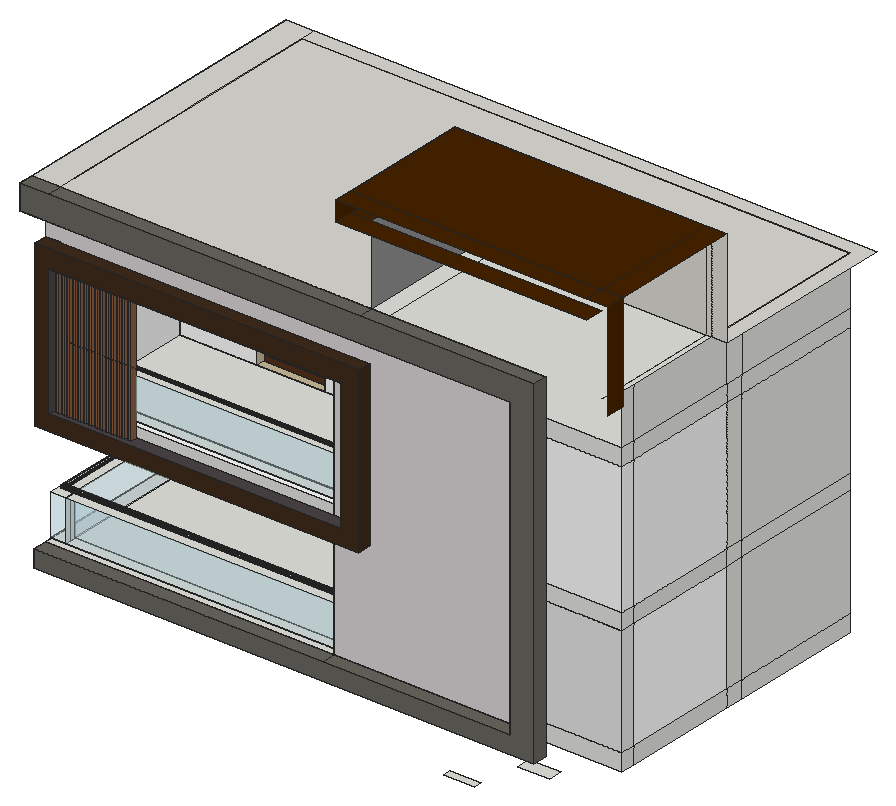
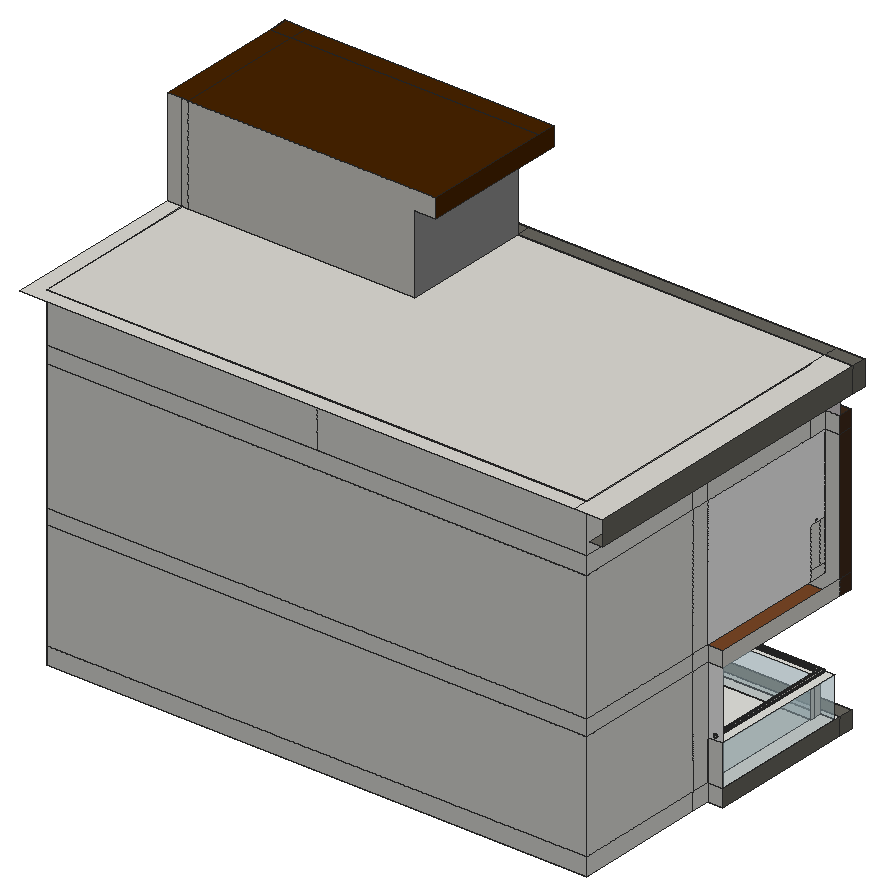
# SketchUp Ruby script. Lengths in inches.
U = 1.inch
M = Sketchup.active_model
def pt(a) = Geom::Point3d.new(a.map { |v| v * U })
def face(e, loops, mat)
  f = e.add_face(loops[0].map { |a| pt(a) })
  loops[1..].each { |l| e.add_face(l.map { |a| pt(a) }).erase! }
  f.material = f.back_material = mat if mat
  f
end
# faces: each face lists its corners as indices into pts; further lists are holes
def faces(e, pts, list, mat = nil) = list.each { |f| face(e, (f[0].is_a?(Array) ? f : [f]).map { |l| l.map { |i| pts[i] } }, mat) }
# xy, xz, yz: faces in a plane at the given z, y or x. An outline is a flat list of corners, or four numbers for a rectangle; further outlines are holes
def ring(l) = l.size == 4 ? [[l[0], l[1]], [l[2], l[1]], [l[2], l[3]], [l[0], l[3]]] : l.each_slice(2).to_a
def flat(e, list, mat, &to3) = list.each { |f| face(e, (f[0].is_a?(Array) ? f : [f]).map { |l| ring(l).map { |u, v| to3.(u, v) } }, mat) }
def xy(e, z, list, mat = nil) = flat(e, list, mat) { |x, y| [x, y, z] }
def xz(e, y, list, mat = nil) = flat(e, list, mat) { |x, z| [x, y, z] }
def yz(e, x, list, mat = nil) = flat(e, list, mat) { |y, z| [x, y, z] }
def lines(e, pts, list) = list.each { |a, b| e.add_line(pt(pts[a]), pt(pts[b])) }
# prism: a flat outline (further loops are holes) pulled along v
def prism(e, loops, v, mat = nil)
  f = face(e, loops, mat); d = Geom::Vector3d.new(v.map { |x| x * U })
  f.pushpull(f.normal.samedirection?(d) ? d.length : -d.length)
end
def box(e, o, s, mat = nil) = prism(e, [[o, [o[0] + s[0], o[1], o[2]], [o[0] + s[0], o[1] + s[1], o[2]], [o[0], o[1] + s[1], o[2]]]], [0, 0, s[2]], mat)
def at(x, y, z, deg = 0) = Geom::Transformation.translation(pt([x, y, z])) * Geom::Transformation.rotation(ORIGIN, Z_AXIS, deg.degrees)
def axes(o, x, y, z) = Geom::Transformation.new([*x, 0, *y, 0, *z, 0, *pt(o).to_a, 1])
def part(name) = M.definitions.add(name)
# library, detail: a bought-in or finely detailed component or shape, given as its bounding box
def library(name, o, s) = part(name).tap { |d| box(d.entities, o, s) }
def detail(e, o, s) = box(e.add_group.entities, o, s)
def put(e, d, t, mat = nil) = e.add_instance(d, t).tap { |i| i.material = mat if mat }
def group(e, t, mat = nil) = e.add_group.tap { |g| g.transformation = t; g.material = mat if mat }.entities
root = M.entities
M.materials.add("[Asphalt New]").color = [76, 68, 70]
M.materials.add("[Blinds Cellular White]").color = [217, 211, 213]
M.materials.add("[Blinds Cellular White]1").color = [217, 211, 213]
M.materials.add("[Carrera Marble]").color = [252, 252, 252]
M.materials.add("[Carrera Marble]1").color = [247, 247, 247]
M.materials.add("[Color C08]").color = [71, 35, 0]
M.materials.add("[Color M01]").color = [226, 226, 226]
M.materials.add("[Color M02]").color = [198, 198, 198]
M.materials.add("[Color M04]").color = [142, 142, 142]
M.materials.add("[Formica Graystone]").color = [104, 102, 94]
M.materials.add("[Quartz Light Brown]").color = [199, 184, 152]
M.materials.add("[Quartz Light Grey]").color = [251, 251, 252]
M.materials.add("[Sandstone]").color = [63, 43, 28]
M.materials.add("[Terrazzo Tile Light]").color = [219, 217, 210]
M.materials.add("[Translucent Glass Safety]").color = [213, 245, 255]
M.materials["[Translucent Glass Safety]"].alpha = 0.35
M.materials.add("[Wood Bamboo]").color = [168, 99, 40]
M.materials.add("[Wood Floor Light]").color = [181, 156, 112]
M.materials.add("[Wood Veneer 01]").color = [84, 49, 25]
M.materials.add("[Wood Veneer 01]1").color = [120, 70, 37]
M.materials.add("[Wood Veneer 02]").color = [140, 94, 67]
xy(root,348.79,[[480.71,442.77,510.46,449.52]])
xy(root,380.34,[[551.08,442.77,580.83,455.77]])
xy(root,382.42,[[190.84,583.41,253.72,588.28]],"[Quartz Light Brown]")
xy(root,382.71,[[295.95,583.41,360.57,591.84]],"[Quartz Light Brown]")
xy(root,397.48,[[118.15,583.41,635.5,601.39],[118.15,601.39,635.5,728.625]])
xy(root,397.48,[[104.01,429.02,376.83,442.77],[376.83,429.02,577.15,442.77]],"[Formica Graystone]")
xy(root,397.48,[[104.01,442.77,104.01,583.41,635.5,583.41,635.5,460.01,376.83,460.01,376.83,442.77]],"[Wood Veneer 01]1")
xy(root,413.92,[[104.01,442.77,376.83,449.27],[104.01,449.27,118.15,583.41],[118.15,449.27,376.83,460.01],[118.15,460.01,635.5,583.41],[118.15,583.41,118.15,601.39,635.5,601.39,635.5,583.41,258.21,583.41,258.21,589.78,192.46,589.78,192.46,583.41],
  [118.15,601.39,635.5,728.625]])
xy(root,413.92,[[104.01,429.02,376.83,442.77],[376.83,429.02,553.9,442.77]],"[Formica Graystone]")
xy(root,413.92,[[192.46,583.41,258.21,589.78]],"[Quartz Light Brown]")
xy(root,434.25,[[289.17,583.41,357.54,594.28]],"[Quartz Light Brown]")
xy(root,452.92,[[104.01,449.27,118.15,583.41],[118.15,449.27,376.83,460.01]])
xy(root,498.23,[[192.46,583.41,258.21,589.78]],"[Quartz Light Brown]")
xy(root,502.625,[[289.17,583.41,357.54,594.28]],"[Quartz Light Brown]")
xy(root,517.48,[[118.15,583.41,635.5,601.39],[118.15,601.39,635.5,728.625]])
xy(root,517.48,[[104.01,429.65,410.58,442.77]],"[Asphalt New]")
xy(root,517.48,[[104.01,442.77,104.01,583.41,635.5,583.41,635.5,460.01,376.83,460.01,376.83,442.77]],"[Wood Veneer 01]1")
xy(root,532.23,[[119.9375,435.4,123.02,441.08],[125.125,435.4,128.2,441.08],[130.3125,435.4,133.39,441.08],[135.5,435.4,138.58,441.08],[140.6875,435.4,143.77,441.08],
  [145.875,435.4,148.95,441.08],[151.0625,435.4,154.14,441.08],[156.25,435.4,159.33,441.08],[161.4375,435.4,164.52,441.08],[166.625,435.4,169.7,441.08],
  [171.8125,435.4,174.89,441.08],[177,435.4,180.08,441.08],[182.1875,435.4,185.27,441.08],[187.375,435.4,190.45,441.08],[118.15,442.77,376.83,460.01],
  [118.15,460.01,635.5,583.41],[118.15,583.41,118.15,601.39,635.5,601.39,635.5,583.41,255.91,583.41,255.91,590.97,191.73,590.97,191.73,583.41],[118.15,601.39,635.5,728.625]])
xy(root,532.23,[[[118.15,429.65,393.7,442.77],[119.9375,435.4,123.02,441.08],[125.125,435.4,128.2,441.08],[130.3125,435.4,133.39,441.08],[135.5,435.4,138.58,441.08],[140.6875,435.4,143.77,441.08],[145.875,435.4,148.95,441.08],[151.0625,435.4,154.14,441.08],[156.25,435.4,159.33,441.08],[161.4375,435.4,164.52,441.08],[166.625,435.4,169.7,441.08],[171.8125,435.4,174.89,441.08],[177,435.4,180.08,441.08],[182.1875,435.4,185.27,441.08],[187.375,435.4,190.45,441.08]]],"[Asphalt New]")
xy(root,532.23,[[191.73,583.41,255.91,590.97]],"[Quartz Light Brown]")
xy(root,553.27,[[286.83,583.41,353,594.78]],"[Quartz Light Brown]")
xy(root,631.6,[[191.73,583.41,255.91,590.97]],"[Quartz Light Brown]")
xy(root,633.96,[[286.83,583.41,353,594.78]],"[Quartz Light Brown]")
xy(root,655.42,[[119.9375,435.4,123.02,441.08]])
xy(root,655.79,[[118.15,583.41,635.5,601.39],[118.15,601.39,635.5,728.625]])
xy(root,655.79,[[[118.15,429.65,118.15,583.41,635.5,583.41,635.5,460.01,376.83,460.01,376.83,442.77,393.7,442.77,393.7,429.65],[125.125,435.4,128.2,441.08],[130.3125,435.4,133.39,441.08],[135.5,435.4,138.58,441.08],[140.6875,435.4,143.77,441.08],[145.875,435.4,148.95,441.08],[151.0625,435.4,154.14,441.08],[156.25,435.4,159.33,441.08],[161.4375,435.4,164.52,441.08],[166.625,435.4,169.7,441.08],[171.8125,435.4,174.89,441.08],[177,435.4,180.08,441.08],[182.1875,435.4,185.27,441.08],[187.375,435.4,190.45,441.08]]],"[Wood Veneer 01]1")
xy(root,672.23,[[118.15,442.77,376.83,728.625],[376.83,460.01,635.5,728.625]])
xy(root,672.23,[[104.01,429.65,410.58,442.77]],"[Sandstone]")
xy(root,695.82,[[91.26,429.02,118.15,442.77],[118.15,429.02,553.9,442.77],[91.26,442.77,104.01,742.77]],"[Formica Graystone]")
xy(root,719.42,[[91.26,429.02,118.15,442.77],[118.15,429.02,412.79,442.77],[412.79,429.02,577.15,442.77]],"[Formica Graystone]")
xy(root,719.42,[[91.26,442.77,118.15,742.77],[118.15,442.77,412.79,442.77,412.79,566.02,635.5,566.02,635.5,728.625,118.15,728.625],[635.5,566.02,649.65,566.02,649.65,742.77,118.15,742.77,118.15,728.625,635.5,728.625]],"[Terrazzo Tile Light]")
xy(root,793.89,[[392.48,424.96,630.01,442.77],[392.48,442.77,412.79,566.02]],"[Color C08]")
xy(root,812.1,[[630.01,424.96,649.65,442.77],[630.01,442.77,649.65,566.02]],"[Color C08]")
xz(root,429.02,[[104.01,397.48,577.15,397.48,577.15,719.42,91.26,719.42,91.26,695.82,553.9,695.82,553.9,413.92,104.01,413.92]],"[Formica Graystone]")
xz(root,429.65,[[[104.01,517.48,410.58,672.23],[118.15,532.23,393.7,655.79]]],"[Sandstone]")
xz(root,435.4,[[119.9375,532.23,123.02,655.42],[125.125,532.23,128.2,655.79],[130.3125,532.23,133.39,655.79],[135.5,532.23,138.58,655.79],[140.6875,532.23,143.77,655.79],
  [145.875,532.23,148.95,655.79],[151.0625,532.23,154.14,655.79],[156.25,532.23,159.33,655.79],[161.4375,532.23,164.52,655.79],[166.625,532.23,169.7,655.79],
  [171.8125,532.23,174.89,655.79],[177,532.23,180.08,655.79],[182.1875,532.23,185.27,655.79],[187.375,532.23,190.45,655.79]],"[Wood Veneer 02]")
xz(root,441.08,[[119.9375,532.23,123.02,655.42],[125.125,532.23,128.2,655.79],[130.3125,532.23,133.39,655.79],[135.5,532.23,138.58,655.79],[140.6875,532.23,143.77,655.79],
  [145.875,532.23,148.95,655.79],[151.0625,532.23,154.14,655.79],[156.25,532.23,159.33,655.79],[161.4375,532.23,164.52,655.79],[166.625,532.23,169.7,655.79],
  [171.8125,532.23,174.89,655.79],[177,532.23,180.08,655.79],[182.1875,532.23,185.27,655.79],[187.375,532.23,190.45,655.79]])
xz(root,442.77,[[104.01,397.48,104.01,413.92,553.9,413.92,553.9,695.82,91.26,695.82,91.26,719.42,577.15,719.42,577.15,397.48],[104.01,517.48,104.01,655.79,118.15,655.79,118.15,532.23,376.83,532.23,376.83,517.48],[376.83,517.48,410.58,517.48,410.58,672.23,393.7,672.23,393.7,532.23,376.83,532.23],[118.15,532.23,376.83,532.23,376.83,541.35,118.15,541.36],[104.01,655.79,118.15,672.23],
  [376.83,655.79,393.7,672.23]])
xz(root,442.77,[[376.83,413.92,553.9,413.92,553.9,695.82,104.01,695.82,104.01,672.23,410.58,672.23,410.58,517.48,376.83,517.48]],"[Blinds Cellular White]")
xz(root,442.77,[[376.83,532.23,393.7,655.79]],"[Blinds Cellular White]1")
xz(root,448.65,[[376.83,541.35,376.83,580.35,118.15,580.36,118.15,541.36]],"[Translucent Glass Safety]")
xz(root,449.27,[[104.01,413.92,118.15,452.92],[118.15,413.92,376.83,452.92]],"[Translucent Glass Safety]")
xz(root,460.01,[[376.83,397.48,635.5,413.92],[376.83,517.48,635.5,532.23],[118.15,532.23,376.83,541.36],[376.83,655.79,635.5,672.23]])
xz(root,460.01,[[376.83,532.23,635.5,655.79]],"[Carrera Marble]1")
xz(root,460.01,[[376.83,413.92,635.5,517.48]],"[Color M01]")
xz(root,460.01,[[118.15,413.92,376.83,452.92],[118.15,541.36,376.83,580.36]],"[Translucent Glass Safety]")
xz(root,566.02,[[412.79,719.42,412.79,793.89,392.48,793.89,392.48,812.11,630.01,812.1,630.01,719.42],[630.01,719.42,635.5,812.1],[635.5,719.42,649.65,812.1]],"[Terrazzo Tile Light]")
xz(root,583.41,[[104.01,397.48,118.15,413.92],[118.15,397.48,635.5,413.92],[104.01,413.92,118.15,452.92],[110.8,454.95,110.3,455.02,109.83,455.21,109.43,455.52,109.12,455.92,108.93,456.39,108.86,456.89,108.93,457.39,109.12,457.86,109.43,458.26,109.83,458.56,110.3,458.76,110.8,458.82,111.3,458.76,111.77,458.56,112.17,458.26,112.48,457.86,112.67,457.39,112.74,456.89,112.67,456.39,112.48,455.92,112.17,455.52,111.77,455.21,111.3,455.02],[104.01,517.48,118.15,532.23],
  [118.15,517.48,635.5,532.23]])
xz(root,583.41,[[[118.15,413.92,192.46,413.92,192.46,498.23,258.21,498.23,258.21,413.92,635.5,413.92,635.5,517.48,118.15,517.48],[289.17,434.25,357.54,502.625]],[[104.01,452.92,118.15,517.48],[110.8,454.95,110.3,455.02,109.83,455.21,109.43,455.52,109.12,455.92,108.93,456.39,108.86,456.89,108.93,457.39,109.12,457.86,109.43,458.26,109.83,458.56,110.3,458.76,110.8,458.82,111.3,458.76,111.77,458.56,112.17,458.26,112.48,457.86,112.67,457.39,112.74,456.89,112.67,456.39,112.48,455.92,112.17,455.52,111.77,455.21,111.3,455.02]],[[118.15,532.23,191.73,532.23,191.73,631.6,255.91,631.6,255.91,532.23,635.5,532.23,635.5,655.79,118.15,655.79],[286.83,553.27,353,633.96]]],"[Carrera Marble]")
xz(root,588.28,[[196.19,345.95,229.61,363.34,228.6,363.69,196.19,374.58],[231.97,364.57,248.36,373.1,248.36,377.07,196.19,377.07]],"[Wood Bamboo]")
xz(root,588.28,[[196.19,342.9,248.36,370.39,248.36,373.1,231.97,364.57,229.61,363.34,196.19,345.95],[229.61,363.34,231.97,364.57,196.19,377.07,196.19,374.58,228.6,363.69]],"[Wood Floor Light]")
xz(root,589.78,[[197.59,419.05,245.43,419.05,197.59,452.25],[253.08,419.05,253.08,443.02,230.22,434.41],[[227.68,436.12,253.08,445.69,253.08,480.75,197.59,460.41,197.59,456.33],[245.76,450.39,248.51,466.08]],[197.59,464.96,228.5625,475.63,197.59,488.63],[231.05,476.48,253.08,484.07,253.08,493.1,197.59,493.1]],"[Wood Bamboo]")
xz(root,589.78,[[245.43,419.05,253.08,419.05,230.22,434.41,227.68,436.12,197.59,456.33,197.59,452.25],[230.22,434.41,253.08,443.02,253.08,445.69,227.68,436.12],[245.76,450.39,248.51,466.08],[197.59,460.41,253.08,480.75,253.08,484.07,231.05,476.48,228.5625,475.63,197.59,464.96],[228.5625,475.63,231.05,476.48,197.59,493.1,197.59,488.63]],"[Wood Floor Light]")
xz(root,589.78,[[[192.46,413.92,258.21,498.23],[197.59,419.05,253.08,493.1]]],"[Wood Veneer 01]")
xz(root,590.97,[[197.78,538.29,243.52,538.29,197.78,580.4],[249.85,538.29,249.85,574.15,229.9,556.02],[[227.81,557.89,249.85,576.58,249.85,615.91,197.78,588.77,197.78,584.59],[241.42,576.58,244.56,594.44]],[197.78,593.1,227.87,607.93,197.78,621.64],[231.99,609.96,249.85,618.77,249.85,625.55,197.78,625.55]],"[Wood Bamboo]")
xz(root,590.97,[[243.52,538.29,249.85,538.29,229.9,556.02,227.81,557.89,197.78,584.59,197.78,580.4],[229.9,556.02,249.85,574.15,249.85,576.58,227.81,557.89],[241.42,576.58,244.56,594.44],[197.78,588.77,249.85,615.91,249.85,618.77,231.99,609.96,227.87,607.93,197.78,593.1],[227.87,607.93,231.99,609.96,197.78,625.55,197.78,621.64]],"[Wood Floor Light]")
xz(root,590.97,[[[191.73,532.23,255.91,631.6],[197.78,538.29,249.85,625.55]]],"[Wood Veneer 01]")
xz(root,594.28,[[293.63,438.71,321.125,498.17],[326.55,438.71,353.09,498.17]],"[Translucent Glass Safety]")
xz(root,594.28,[[[289.17,434.25,357.54,502.625],[293.63,438.71,353.09,498.17]],[321.125,438.71,326.55,498.17]],"[Wood Veneer 01]")
xz(root,594.78,[[292.52,558.96,317.19,628.28],[322.88,558.96,347.32,628.28]],"[Translucent Glass Safety]")
xz(root,594.78,[[[286.83,553.27,353,633.96],[292.52,558.96,347.32,628.28]],[317.19,558.96,322.88,628.28]],"[Wood Veneer 01]")
xz(root,601.39,[[118.15,397.48,635.5,413.92],[118.15,413.92,635.5,517.48],[118.15,517.48,635.5,532.23],[118.15,532.23,635.5,655.79]])
xz(root,728.625,[[118.15,397.48,635.5,413.92],[118.15,413.92,635.5,517.48],[118.15,517.48,635.5,532.23],[118.15,532.23,635.5,655.79],[118.15,655.79,635.5,672.23],
  [118.15,672.23,376.83,719.42],[376.83,672.23,635.5,719.42]])
yz(root,91.26,[[429.02,695.82,442.77,719.42],[442.77,695.82,742.77,719.42]],"[Formica Graystone]")
yz(root,104.01,[[429.02,397.48,442.77,413.92],[442.77,397.48,583.41,413.92]],"[Formica Graystone]")
yz(root,104.01,[[429.65,517.48,442.77,532.23],[429.65,532.23,442.77,655.79],[429.65,655.79,442.77,672.23]],"[Sandstone]")
yz(root,104.01,[[442.77,517.48,583.41,532.23]],"[Terrazzo Tile Light]")
yz(root,104.01,[[449.27,413.92,583.41,452.92]],"[Translucent Glass Safety]")
yz(root,118.15,[[583.41,397.48,601.39,413.92],[601.39,397.48,728.625,413.92],[449.27,413.92,455.34,452.92],[455.34,413.92,460.01,452.92],[583.41,413.92,601.39,517.48],
  [601.39,413.92,728.625,517.48],[583.41,517.48,601.39,532.23],[601.39,517.48,728.625,532.23],[442.77,532.23,460.01,541.36],[583.41,532.23,601.39,655.79],
  [601.39,532.23,728.625,655.79],[442.77,541.36,448.65,580.36],[448.65,541.36,460.01,580.36],[454.28,581.7,453.96,581.74,453.65,581.87,453.39,582.0625,453.2,582.32,453.07,582.625,453.03,582.95,453.07,583.27,453.2,583.57,453.39,583.83,453.65,584.03,453.96,584.16,454.28,584.2,454.6,584.16,454.9,584.03,455.16,583.83,455.36,583.57,455.49,583.27,455.53,582.95,455.49,582.625,455.36,582.32,455.16,582.0625,454.9,581.87,454.6,581.74],[442.77,655.79,460.01,672.23],
  [460.01,655.79,583.41,672.23],[583.41,655.79,601.39,672.23],[601.39,655.79,728.625,672.23],[460.01,672.23,583.41,719.42],[583.41,672.23,601.39,719.42],
  [601.39,672.23,728.625,719.42]])
yz(root,118.15,[[429.65,532.23,442.77,655.79]],"[Asphalt New]")
yz(root,118.15,[[[460.01,532.23,583.41,532.23,583.41,655.79,442.77,655.79,442.77,580.36,460.01,580.36],[454.28,581.7,453.96,581.74,453.65,581.87,453.39,582.0625,453.2,582.32,453.07,582.625,453.03,582.95,453.07,583.27,453.2,583.57,453.39,583.83,453.65,584.03,453.96,584.16,454.28,584.2,454.6,584.16,454.9,584.03,455.16,583.83,455.36,583.57,455.49,583.27,455.53,582.95,455.49,582.625,455.36,582.32,455.16,582.0625,454.9,581.87,454.6,581.74]]],"[Carrera Marble]1")
yz(root,118.15,[[460.01,413.92,583.41,452.92]],"[Translucent Glass Safety]")
yz(root,119.9375,[[435.4,532.23,441.08,655.42]])
yz(root,123.02,[[435.4,532.23,441.08,655.42]],"[Wood Veneer 02]")
yz(root,125.125,[[435.4,532.23,441.08,655.79]],"[Wood Veneer 02]")
yz(root,128.2,[[435.4,532.23,441.08,655.79]],"[Wood Veneer 02]")
yz(root,130.3125,[[435.4,532.23,441.08,655.79]],"[Wood Veneer 02]")
yz(root,133.39,[[435.4,532.23,441.08,655.79]],"[Wood Veneer 02]")
yz(root,135.5,[[435.4,532.23,441.08,655.79]],"[Wood Veneer 02]")
yz(root,138.58,[[435.4,532.23,441.08,655.79]],"[Wood Veneer 02]")
yz(root,140.6875,[[435.4,532.23,441.08,655.79]],"[Wood Veneer 02]")
yz(root,143.77,[[435.4,532.23,441.08,655.79]],"[Wood Veneer 02]")
yz(root,145.875,[[435.4,532.23,441.08,655.79]],"[Wood Veneer 02]")
yz(root,148.95,[[435.4,532.23,441.08,655.79]],"[Wood Veneer 02]")
yz(root,151.0625,[[435.4,532.23,441.08,655.79]],"[Wood Veneer 02]")
yz(root,154.14,[[435.4,532.23,441.08,655.79]],"[Wood Veneer 02]")
yz(root,156.25,[[435.4,532.23,441.08,655.79]],"[Wood Veneer 02]")
yz(root,159.33,[[435.4,532.23,441.08,655.79]],"[Wood Veneer 02]")
yz(root,161.4375,[[435.4,532.23,441.08,655.79]],"[Wood Veneer 02]")
yz(root,164.52,[[435.4,532.23,441.08,655.79]],"[Wood Veneer 02]")
yz(root,166.625,[[435.4,532.23,441.08,655.79]],"[Wood Veneer 02]")
yz(root,169.7,[[435.4,532.23,441.08,655.79]],"[Wood Veneer 02]")
yz(root,171.8125,[[435.4,532.23,441.08,655.79]],"[Wood Veneer 02]")
yz(root,174.89,[[435.4,532.23,441.08,655.79]],"[Wood Veneer 02]")
yz(root,177,[[435.4,532.23,441.08,655.79]],"[Wood Veneer 02]")
yz(root,180.08,[[435.4,532.23,441.08,655.79]],"[Wood Veneer 02]")
yz(root,182.1875,[[435.4,532.23,441.08,655.79]],"[Wood Veneer 02]")
yz(root,185.27,[[435.4,532.23,441.08,655.79]],"[Wood Veneer 02]")
yz(root,187.375,[[435.4,532.23,441.08,655.79]],"[Wood Veneer 02]")
yz(root,190.45,[[435.4,532.23,441.08,655.79]],"[Wood Veneer 02]")
yz(root,191.73,[[583.41,532.23,590.97,631.6]],"[Quartz Light Brown]")
yz(root,192.46,[[583.41,413.92,589.78,498.23]],"[Quartz Light Brown]")
yz(root,255.91,[[583.41,532.23,590.97,631.6]],"[Quartz Light Brown]")
yz(root,258.21,[[583.41,413.92,589.78,498.23]],"[Quartz Light Brown]")
yz(root,286.83,[[583.41,553.27,594.78,633.96]],"[Quartz Light Brown]")
yz(root,289.17,[[583.41,434.25,594.28,502.625]],"[Quartz Light Brown]")
yz(root,353,[[583.41,553.27,594.78,633.96]],"[Quartz Light Brown]")
yz(root,357.54,[[583.41,434.25,594.28,502.625]],"[Quartz Light Brown]")
yz(root,376.83,[[449.27,413.92,460.01,452.92],[442.77,517.48,460.01,532.23],[442.77,532.23,442.77,541.35,448.65,541.35,460.01,541.36,460.01,532.23],[442.77,541.35,448.65,580.35],[448.65,541.35,448.65,580.35,460.01,580.36,460.01,541.36],
  [442.77,655.79,460.01,672.23]])
yz(root,376.83,[[[442.77,413.92,442.77,517.48,460.01,517.48,460.01,452.92,449.27,452.92,449.27,413.92],[456.78,454.95,457.28,455.02,457.75,455.21,458.15,455.52,458.46,455.92,458.65,456.39,458.72,456.89,458.65,457.39,458.46,457.86,458.15,458.26,457.75,458.56,457.28,458.76,456.78,458.82,456.28,458.76,455.8125,458.56,455.41,458.26,455.1,457.86,454.91,457.39,454.84,456.89,454.91,456.39,455.1,455.92,455.41,455.52,455.8125,455.21,456.28,455.02]],[[442.77,580.35,442.77,655.79,460.01,655.79,460.01,580.36,448.65,580.35],[454.28,581.7,454.6,581.74,454.9,581.87,455.16,582.0625,455.36,582.32,455.49,582.625,455.53,582.95,455.49,583.27,455.36,583.57,455.16,583.83,454.9,584.03,454.6,584.16,454.28,584.2,453.96,584.16,453.65,584.03,453.39,583.83,453.2,583.57,453.07,583.27,453.03,582.95,453.07,582.625,453.2,582.32,453.39,582.0625,453.65,581.87,453.96,581.74]]],"[Color M02]")
yz(root,392.48,[[424.96,793.89,424.96,812.1,442.77,812.11,566.02,812.11,566.02,793.89]],"[Color C08]")
yz(root,393.7,[[429.65,532.23,442.77,655.79]],"[Asphalt New]")
yz(root,410.58,[[429.65,517.48,442.77,655.79],[429.65,655.79,442.77,672.23]],"[Sandstone]")
yz(root,412.79,[[442.77,719.42,566.02,793.89]],"[Color M04]")
yz(root,553.9,[[429.02,413.92,442.77,695.82]],"[Formica Graystone]")
yz(root,577.15,[[429.02,397.48,442.77,719.42]],"[Formica Graystone]")
yz(root,635.5,[[460.01,397.48,474.16,413.92],[474.16,397.48,583.41,413.92],[583.41,397.48,601.39,413.92],[601.39,397.48,728.625,413.92],[583.41,413.92,601.39,517.48],
  [601.39,413.92,728.625,517.48],[460.01,517.48,474.16,532.23],[474.16,517.48,583.41,532.23],[583.41,517.48,601.39,532.23],[601.39,517.48,728.625,532.23],
  [583.41,532.23,601.39,655.79],[601.39,532.23,728.625,655.79],[460.01,655.79,474.16,672.23],[474.16,655.79,583.41,672.23],[583.41,655.79,601.39,672.23],
  [601.39,655.79,728.625,672.23],[460.01,672.23,474.16,719.42],[474.16,672.23,583.41,719.42],[583.41,672.23,601.39,719.42],[601.39,672.23,728.625,719.42]])
yz(root,635.5,[[474.16,413.92,583.41,517.48]],"[Carrera Marble]")
yz(root,635.5,[[460.01,532.23,474.16,655.79],[474.16,532.23,583.41,655.79]],"[Carrera Marble]1")
yz(root,635.5,[[460.01,413.92,474.16,517.48]],"[Color M01]")
yz(root,649.65,[[424.96,719.42,442.77,812.1]],"[Color C08]")
p = [[110.3,583.41,455.02],[110.8,583.41,454.95],[110.8,456.78,454.95],[110.3,456.28,455.02],[376.83,456.78,454.95],[376.83,456.28,455.02],
  [111.3,583.41,455.02],[111.3,457.28,455.02],[376.83,457.28,455.02],[109.83,583.41,455.21],[109.83,455.8125,455.21],[376.83,455.8125,455.21],
  [111.77,583.41,455.21],[111.77,457.75,455.21],[376.83,457.75,455.21],[109.43,583.41,455.52],[109.43,455.41,455.52],[376.83,455.41,455.52],
  [112.17,583.41,455.52],[112.17,458.15,455.52],[376.83,458.15,455.52],[109.12,583.41,455.92],[109.12,455.1,455.92],[376.83,455.1,455.92],
  [112.48,583.41,455.92],[112.48,458.46,455.92],[376.83,458.46,455.92],[108.93,583.41,456.39],[108.93,454.91,456.39],[376.83,454.91,456.39],
  [112.67,583.41,456.39],[112.67,458.65,456.39],[376.83,458.65,456.39],[108.86,583.41,456.89],[108.86,454.84,456.89],[376.83,454.84,456.89],
  [112.74,583.41,456.89],[112.74,458.72,456.89],[376.83,458.72,456.89],[108.93,583.41,457.39],[108.93,454.91,457.39],[376.83,454.91,457.39],
  [112.67,583.41,457.39],[112.67,458.65,457.39],[376.83,458.65,457.39],[109.12,583.41,457.86],[109.12,455.1,457.86],[376.83,455.1,457.86],
  [112.48,583.41,457.86],[112.48,458.46,457.86],[376.83,458.46,457.86],[109.43,583.41,458.26],[109.43,455.41,458.26],[376.83,455.41,458.26],
  [112.17,583.41,458.26],[112.17,458.15,458.26],[376.83,458.15,458.26],[109.83,583.41,458.56],[109.83,455.8125,458.56],[376.83,455.8125,458.56],
  [111.77,583.41,458.56],[111.77,457.75,458.56],[376.83,457.75,458.56],[110.3,583.41,458.76],[110.3,456.28,458.76],[376.83,456.28,458.76],
  [111.3,583.41,458.76],[111.3,457.28,458.76],[376.83,457.28,458.76],[110.8,583.41,458.82],[110.8,456.78,458.82],[376.83,456.78,458.82],
  [376.83,442.77,541.35],[118.15,442.77,541.36],[118.15,448.65,541.36],[376.83,448.65,541.35],[376.83,460.01,541.36],[118.15,460.01,541.36],
  [376.83,448.65,580.35],[376.83,460.01,580.36],[118.15,460.01,580.36],[118.15,448.65,580.36],[118.15,453.65,581.87],[118.15,453.96,581.74],
  [376.83,453.96,581.74],[376.83,453.65,581.87],[118.15,454.28,581.7],[376.83,454.28,581.7],[118.15,454.6,581.74],[376.83,454.6,581.74],
  [118.15,454.9,581.87],[376.83,454.9,581.87],[118.15,453.39,582.0625],[376.83,453.39,582.0625],[118.15,455.16,582.0625],[376.83,455.16,582.0625],
  [118.15,453.2,582.32],[376.83,453.2,582.32],[118.15,455.36,582.32],[376.83,455.36,582.32],[118.15,453.07,582.625],[376.83,453.07,582.625],
  [118.15,455.49,582.625],[376.83,455.49,582.625],[118.15,453.03,582.95],[376.83,453.03,582.95],[118.15,455.53,582.95],[376.83,455.53,582.95],
  [118.15,453.07,583.27],[376.83,453.07,583.27],[118.15,455.49,583.27],[376.83,455.49,583.27],[118.15,453.2,583.57],[376.83,453.2,583.57],
  [118.15,455.36,583.57],[376.83,455.36,583.57],[118.15,453.39,583.83],[376.83,453.39,583.83],[118.15,455.16,583.83],[376.83,455.16,583.83],
  [118.15,453.65,584.03],[376.83,453.65,584.03],[118.15,454.9,584.03],[376.83,454.9,584.03],[118.15,453.96,584.16],[376.83,453.96,584.16],
  [118.15,454.6,584.16],[376.83,454.6,584.16],[118.15,454.28,584.2],[376.83,454.28,584.2],[630.01,442.77,812.1],[392.48,442.77,812.11],
  [392.48,424.96,812.1],[630.01,424.96,812.1],[630.01,566.02,812.1],[392.48,566.02,812.11],[110.8,583.41,456.89],[110.8,456.78,456.89],
  [376.83,456.78,456.89],[630.01,566.02,719.42],[630.01,442.77,719.42]]
faces(root,p,[[0,1,2,3],[3,2,4,5],[1,6,7,2],[2,7,8,4],[9,0,3,10],[10,3,5,11],[6,12,13,7],[7,13,14,8],
  [15,9,10,16],[16,10,11,17],[12,18,19,13],[13,19,20,14],[21,15,16,22],[22,16,17,23],[18,24,25,19],[19,25,26,20],
  [27,21,22,28],[28,22,23,29],[24,30,31,25],[25,31,32,26],[33,27,28,34],[34,28,29,35],[30,36,37,31],[31,37,38,32],
  [39,33,34,40],[40,34,35,41],[36,42,43,37],[37,43,44,38],[45,39,40,46],[46,40,41,47],[42,48,49,43],[43,49,50,44],
  [51,45,46,52],[52,46,47,53],[48,54,55,49],[49,55,56,50],[57,51,52,58],[58,52,53,59],[54,60,61,55],[55,61,62,56],
  [63,57,58,64],[64,58,59,65],[60,66,67,61],[61,67,68,62],[69,63,64,70],[70,64,65,71],[66,69,70,67],[67,70,71,68],
  [82,83,84,85],[83,86,87,84],[86,88,89,87],[88,90,91,89],[92,82,85,93],[90,94,95,91],[96,92,93,97],[94,98,99,95],
  [100,96,97,101],[98,102,103,99],[104,100,101,105],[102,106,107,103],[108,104,105,109],[106,110,111,107],[112,108,109,113],[110,114,115,111],
  [116,112,113,117],[114,118,119,115],[120,116,117,121],[118,122,123,119],[124,120,121,125],[122,126,127,123],[128,124,125,129],[126,128,129,127]],"[Terrazzo Tile Light]")
faces(root,p,[[72,73,74,75]],"[Quartz Light Grey]")
faces(root,p,[[76,75,74,77],[78,79,80,81]])
faces(root,p,[[130,131,132,133],[130,134,135,131]],"[Color C08]")
lines(root,p,[[136,137],[137,138],[139,140]])
